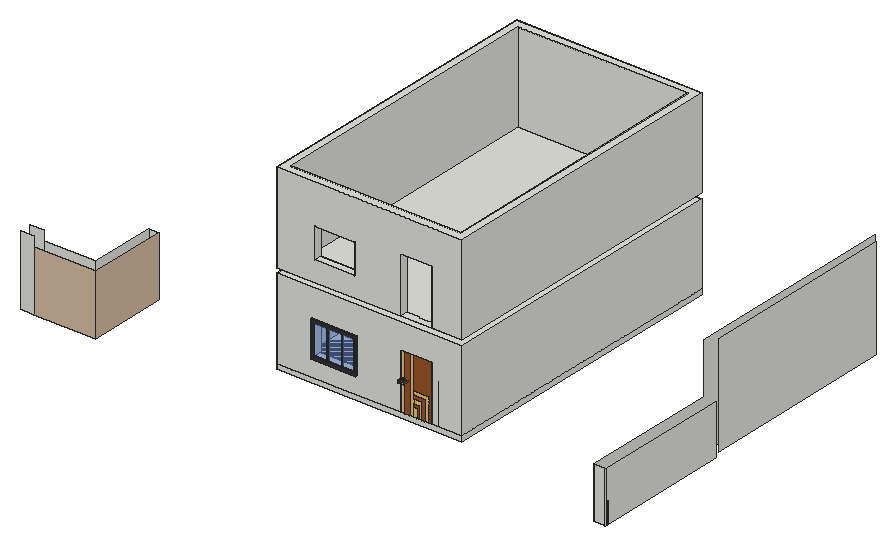
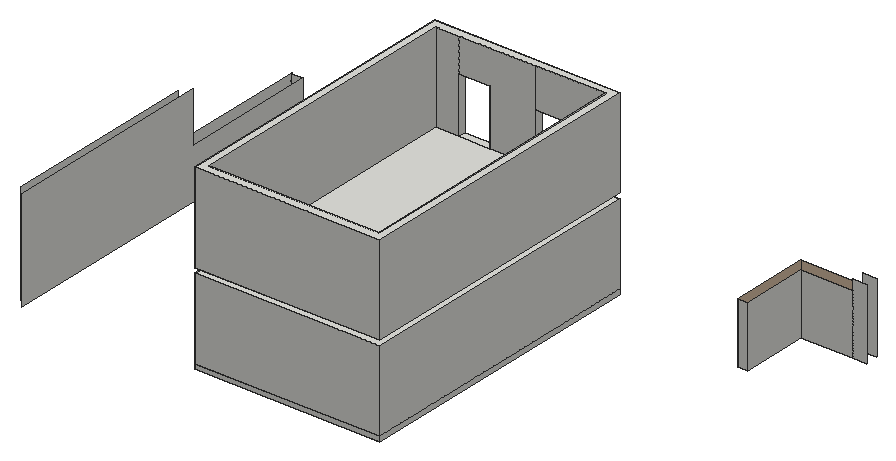
# SketchUp Ruby script. Lengths in inches.
U = 1.inch
M = Sketchup.active_model
def pt(a) = Geom::Point3d.new(a.map { |v| v * U })
def face(e, loops, mat)
  f = e.add_face(loops[0].map { |a| pt(a) })
  loops[1..].each { |l| e.add_face(l.map { |a| pt(a) }).erase! }
  f.material = f.back_material = mat if mat
  f
end
# faces: each face lists its corners as indices into pts; further lists are holes
def faces(e, pts, list, mat = nil) = list.each { |f| face(e, (f[0].is_a?(Array) ? f : [f]).map { |l| l.map { |i| pts[i] } }, mat) }
# xy, xz, yz: faces in a plane at the given z, y or x. An outline is a flat list of corners, or four numbers for a rectangle; further outlines are holes
def ring(l) = l.size == 4 ? [[l[0], l[1]], [l[2], l[1]], [l[2], l[3]], [l[0], l[3]]] : l.each_slice(2).to_a
def flat(e, list, mat, &to3) = list.each { |f| face(e, (f[0].is_a?(Array) ? f : [f]).map { |l| ring(l).map { |u, v| to3.(u, v) } }, mat) }
def xy(e, z, list, mat = nil) = flat(e, list, mat) { |x, y| [x, y, z] }
def xz(e, y, list, mat = nil) = flat(e, list, mat) { |x, z| [x, y, z] }
def yz(e, x, list, mat = nil) = flat(e, list, mat) { |y, z| [x, y, z] }
def lines(e, pts, list) = list.each { |a, b| e.add_line(pt(pts[a]), pt(pts[b])) }
# prism: a flat outline (further loops are holes) pulled along v
def prism(e, loops, v, mat = nil)
  f = face(e, loops, mat); d = Geom::Vector3d.new(v.map { |x| x * U })
  f.pushpull(f.normal.samedirection?(d) ? d.length : -d.length)
end
def box(e, o, s, mat = nil) = prism(e, [[o, [o[0] + s[0], o[1], o[2]], [o[0] + s[0], o[1] + s[1], o[2]], [o[0], o[1] + s[1], o[2]]]], [0, 0, s[2]], mat)
def at(x, y, z, deg = 0) = Geom::Transformation.translation(pt([x, y, z])) * Geom::Transformation.rotation(ORIGIN, Z_AXIS, deg.degrees)
def axes(o, x, y, z) = Geom::Transformation.new([*x, 0, *y, 0, *z, 0, *pt(o).to_a, 1])
def part(name) = M.definitions.add(name)
# library, detail: a bought-in or finely detailed component or shape, given as its bounding box
def library(name, o, s) = part(name).tap { |d| box(d.entities, o, s) }
def detail(e, o, s) = box(e.add_group.entities, o, s)
def put(e, d, t, mat = nil) = e.add_instance(d, t).tap { |i| i.material = mat if mat }
def group(e, t, mat = nil) = e.add_group.tap { |g| g.transformation = t; g.material = mat if mat }.entities
root = M.entities
M.materials.add("[Formica Laminate Dark]").color = [50, 53, 60]
M.materials.add("[Formica Laminate Light]").color = [213, 189, 164]
M.materials.add("[Translucent Glass Blue]").color = [100, 149, 237]
M.materials["[Translucent Glass Blue]"].alpha = 0.5
M.materials.add("[Wood Cherry Original]").color = [152, 86, 42]
M.materials.add("[Wood OSB]").color = [240, 195, 122]
xy(root,-4.7,[[671.44,112.73,890.94,467.89]])
xy(root,0,[[1084.25,65.97,1098.46,88.97],[1084.25,88.97,1098.46,229.27]])
xy(root,1.3,[[671.44,112.73,890.94,467.89]])
xy(root,21.73,[[713.56,110.73,766.93,112.73]],"[Formica Laminate Dark]")
xy(root,25.3,[[732.16,111.73,733.7,112.73],[748.89,111.73,750.4,112.73]])
xy(root,25.3,[[716.85,110.73,764.09,110.73,764.09,112.73,750.4,112.73,750.4,111.73,748.89,111.73,748.89,112.73,733.7,112.73,733.7,111.73,732.16,111.73,732.16,112.73,716.85,112.73]],"[Formica Laminate Dark]")
xy(root,36.23,[[822.16,107.04,826.99,112.73]],"[Wood Cherry Original]")
xy(root,37.73,[[822.16,107.04,826.99,112.73]],"[Wood Cherry Original]")
xy(root,61.3,[[716.85,110.73,716.85,112.73,732.16,112.73,732.16,111.73,733.7,111.73,733.7,112.73,748.89,112.73,748.89,111.73,750.4,111.73,750.4,112.73,764.09,112.73,764.09,110.73],[732.16,111.73,733.7,112.73],[748.89,111.73,750.4,112.73]])
xy(root,64.36,[[713.56,110.73,766.93,112.73]],"[Formica Laminate Dark]")
xz(root,54.73,[[414.0625,-6,429.79,77.75]])
xz(root,54.73,[[429.79,-6,503.53,65.8125]],"[Formica Laminate Light]")
xz(root,65.97,[[1084.25,0,1098.46,60]])
xz(root,69.27,[[414.0625,-6,429.79,77.75],[429.79,-6,491.63,65.8125]])
xz(root,107.04,[[820.87,35.48,821.25,35.53,821.62,35.68,821.93,35.92,822.16,36.23,826.99,36.23,826.99,37.73,822.16,37.73,821.93,38.04,821.62,38.27,821.25,38.42,820.87,38.48,820.48,38.42,820.12,38.27,819.8,38.04,819.57,37.73,819.42,37.36,819.37,36.98,819.42,36.59,819.57,36.23,819.8,35.92,820.12,35.68,820.48,35.53]],"[Wood OSB]")
xz(root,110.73,[[[713.56,21.73,766.93,64.36],[716.85,25.3,764.09,61.3]]],"[Formica Laminate Dark]")
xz(root,111.73,[[732.16,25.3,733.7,61.3],[748.89,25.3,750.4,61.3]],"[Formica Laminate Dark]")
xz(root,112.73,[[671.44,-4.7,890.94,1.3],[[713.56,21.73,766.93,64.36],[716.85,25.3,764.09,61.3]]])
xz(root,112.73,[[716.85,25.3,732.16,61.3],[733.7,25.3,748.89,61.3],[750.4,25.3,764.09,61.3]],"[Translucent Glass Blue]")
xz(root,112.73,[[823.38,1.3,828.92,1.3,828.92,67.3,823.38,67.3,823.38,37.73,826.99,37.73,826.99,36.23,823.38,36.23],[837.11,1.3,839.55,1.3,839.55,15.69,833.55,15.69,833.55,11.92,837.11,11.92],[843.11,1.3,847.23,1.3,847.23,24.66,833.55,24.66,833.55,20.72,843.11,20.72],[851.86,1.3,854.85,1.3,854.85,67.3,833.55,67.3,833.55,29.63,851.86,29.63]],"[Wood Cherry Original]")
xz(root,112.73,[[818.26,1.3,823.38,1.3,823.38,36.23,822.16,36.23,821.93,35.92,821.62,35.68,821.25,35.53,820.87,35.48,820.48,35.53,820.12,35.68,819.8,35.92,819.57,36.23,819.42,36.59,819.37,36.98,819.42,37.36,819.57,37.73,819.8,38.04,820.12,38.27,820.48,38.42,820.87,38.48,821.25,38.42,821.62,38.27,821.93,38.04,822.16,37.73,823.38,37.73,823.38,67.3,818.26,67.3],[828.92,1.3,833.55,67.3],[833.55,1.3,837.11,11.92],[839.55,1.3,843.11,1.3,843.11,20.72,833.55,20.72,833.55,15.69,839.55,15.69],[847.23,1.3,851.86,1.3,851.86,29.63,833.55,29.63,833.55,24.66,847.23,24.66]],"[Wood OSB]")
xz(root,148.73,[[491.63,-6,503.53,65.8125]])
xz(root,467.89,[[671.44,-4.7,890.94,1.3]])
yz(root,491.63,[[69.27,-6,148.73,65.8125]])
yz(root,503.53,[[54.73,-6,148.73,65.8125]],"[Formica Laminate Light]")
yz(root,671.44,[[112.73,-4.7,467.89,1.3]])
yz(root,713.56,[[110.73,21.73,112.73,64.36]],"[Formica Laminate Dark]")
yz(root,716.85,[[110.73,25.3,112.73,61.3]],"[Formica Laminate Dark]")
yz(root,732.16,[[111.73,25.3,112.73,61.3]],"[Formica Laminate Dark]")
yz(root,733.7,[[111.73,25.3,112.73,61.3]],"[Formica Laminate Dark]")
yz(root,748.89,[[111.73,25.3,112.73,61.3]],"[Formica Laminate Dark]")
yz(root,750.4,[[111.73,25.3,112.73,61.3]],"[Formica Laminate Dark]")
yz(root,764.09,[[110.73,25.3,112.73,61.3]],"[Formica Laminate Dark]")
yz(root,766.93,[[110.73,21.73,112.73,64.36]],"[Formica Laminate Dark]")
yz(root,826.99,[[107.04,36.23,112.73,37.73]],"[Wood Cherry Original]")
yz(root,890.94,[[112.73,-4.7,467.89,1.3]])
yz(root,1084.25,[[65.97,0,65.97,60,229.27,60,229.27,120,482.79,120,482.79,0]])
yz(root,1093.25,[[240.05,0,473.79,120]])
yz(root,1098.46,[[64.97,0,65.97,60],[65.97,0,229.27,60]])
yz(root,1101.82,[[64.97,3.36,65.97,5.49],[64.97,5.49,65.97,5.5],[64.97,5.5,65.97,7.62],[64.97,7.62,65.97,7.63],[64.97,7.63,65.97,9.75],
  [64.97,9.75,65.97,9.76],[64.97,9.76,65.97,11.88],[64.97,11.88,65.97,11.9],[64.97,11.9,65.97,14.01],[64.97,14.01,65.97,14.03],
  [64.97,14.03,65.97,16.14],[64.97,16.14,65.97,16.16],[64.97,16.16,65.97,18.27],[64.97,18.27,65.97,18.29],[64.97,18.29,65.97,20.4],
  [64.97,20.4,65.97,20.42],[64.97,20.42,65.97,22.53],[64.97,22.53,65.97,22.55],[64.97,22.55,65.97,24.66],[64.97,24.66,65.97,24.68],
  [64.97,24.68,65.97,26.8],[64.97,26.8,65.97,26.8125]])
p = [[820.12,112.73,35.68],[820.48,112.73,35.53],[820.48,107.04,35.53],[820.12,107.04,35.68],[820.87,112.73,35.48],[820.87,107.04,35.48],
  [821.25,112.73,35.53],[821.25,107.04,35.53],[821.62,112.73,35.68],[821.62,107.04,35.68],[819.8,112.73,35.92],[819.8,107.04,35.92],
  [821.93,112.73,35.92],[821.93,107.04,35.92],[819.57,112.73,36.23],[819.57,107.04,36.23],[822.16,112.73,36.23],[822.16,107.04,36.23],
  [819.42,112.73,36.59],[819.42,107.04,36.59],[819.37,112.73,36.98],[819.37,107.04,36.98],[819.42,112.73,37.36],[819.42,107.04,37.36],
  [819.57,112.73,37.73],[819.57,107.04,37.73],[819.8,112.73,38.04],[819.8,107.04,38.04],[822.16,112.73,37.73],[821.93,112.73,38.04],
  [821.93,107.04,38.04],[822.16,107.04,37.73],[820.12,112.73,38.27],[820.12,107.04,38.27],[821.62,112.73,38.27],[821.62,107.04,38.27],
  [820.48,112.73,38.42],[820.48,107.04,38.42],[821.25,112.73,38.42],[821.25,107.04,38.42],[820.87,112.73,38.48],[820.87,107.04,38.48],
  [862.5,112.73,1.3],[862.5,112.73,49.3]]
faces(root,p,[[0,1,2,3],[1,4,5,2],[4,6,7,5],[6,8,9,7],[10,0,3,11],[8,12,13,9],[14,10,11,15],[12,16,17,13],
  [18,14,15,19],[20,18,19,21],[22,20,21,23],[24,22,23,25],[26,24,25,27],[28,29,30,31],[32,26,27,33],[29,34,35,30],
  [36,32,33,37],[34,38,39,35],[40,36,37,41],[38,40,41,39]],"[Wood OSB]")
lines(root,p,[[42,43]])
g1 = group(root,at(671.44,112.73,1.3))
xy(g1,0,[[0,0,92.65,0,92.65,9,9,9,9,346.16,210.5,346.16,210.5,9,183.41,9,183.41,0,219.5,0,219.5,355.16,0,355.16],[146.8125,0,183.41,9],[9,9,210.5,346.16]])
xy(g1,24,[[45.41,0,92.65,9]])
xy(g1,60,[[45.41,0,92.65,9]])
xy(g1,66,[[146.8125,0,183.41,9]])
xy(g1,96,[[[0,0,219.5,355.16],[9,9,210.5,346.16]]])
xy(g1,102,[[0,0,92.65,0,92.65,9,9,9,9,346.16,210.5,346.16,210.5,9,183.41,9,183.41,0,219.5,0,219.5,355.16,0,355.16],[146.8125,0,183.41,9],[9,9,210.5,346.16]])
xy(g1,126,[[45.41,0,92.65,9]])
xy(g1,162,[[45.41,0,92.65,9]])
xy(g1,168,[[146.8125,0,183.41,9]])
xy(g1,208.9375,[[[0,0,219.5,355.16],[9,9,210.5,346.16]]])
xz(g1,0,[[[0,0,146.8125,0,146.8125,66,183.41,66,183.41,0,219.5,0,219.5,96,0,96],[45.41,24,92.65,60]],[[0,102,146.8125,102,146.8125,168,183.41,168,183.41,102,219.5,102,219.5,208.9375,0,208.9375],[45.41,126,92.65,162]]])
xz(g1,9,[[9,0,9,96,92.65,96,92.65,60,45.41,60,45.41,24,92.65,24,92.65,0],[92.65,0,92.65,96,183.41,96,183.41,66,146.8125,66,146.8125,0],[183.41,0,210.5,96],[9,102,9,208.9375,92.65,208.9375,92.65,162,45.41,162,45.41,126,92.65,126,92.65,102],[92.65,102,92.65,208.9375,183.41,208.9375,183.41,168,146.8125,168,146.8125,102],
  [183.41,102,210.5,208.9375]])
xz(g1,346.16,[[9,0,210.5,96],[9,102,210.5,208.9375]])
xz(g1,355.16,[[0,0,219.5,96],[0,102,219.5,208.9375]])
yz(g1,0,[[0,0,355.16,96],[0,102,355.16,208.9375]])
yz(g1,9,[[9,0,346.16,96],[9,102,346.16,208.9375]])
yz(g1,45.41,[[0,24,9,60],[0,126,9,162]])
yz(g1,92.65,[[0,24,9,60],[0,126,9,162]])
yz(g1,146.8125,[[0,0,9,66],[0,102,9,168]])
yz(g1,183.41,[[0,0,9,66],[0,102,9,168]])
yz(g1,210.5,[[9,0,346.16,96],[9,102,346.16,208.9375]])
yz(g1,219.5,[[0,0,355.16,96],[0,102,355.16,208.9375]])
